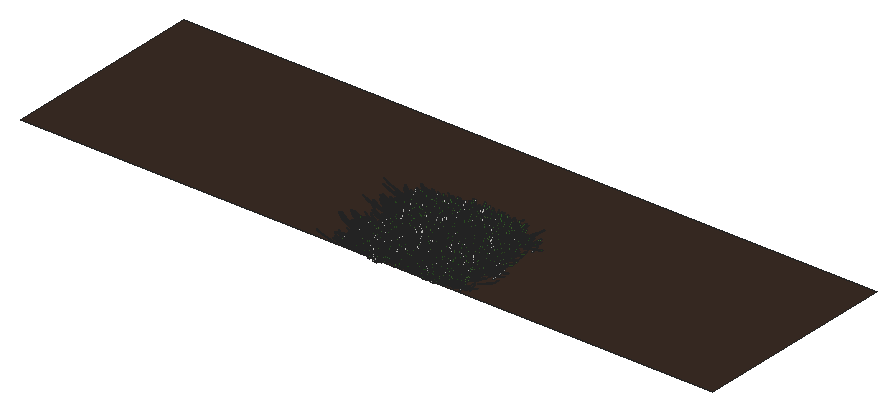
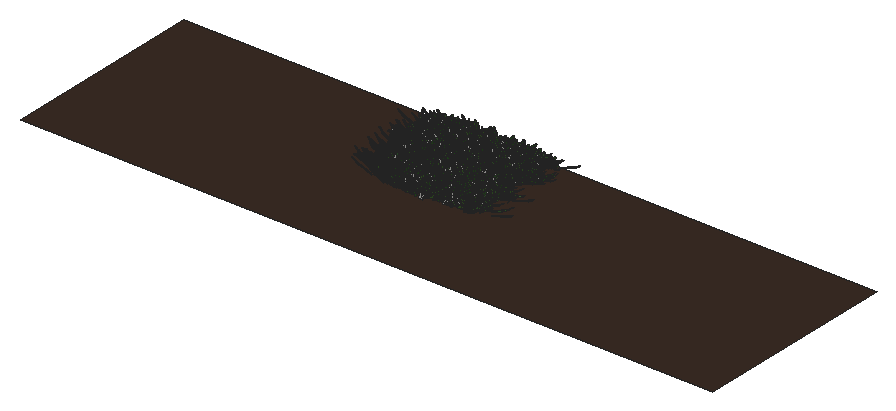
# SketchUp Ruby script. Lengths in inches.
U = 1.inch
M = Sketchup.active_model
def pt(a) = Geom::Point3d.new(a.map { |v| v * U })
def face(e, loops, mat)
  f = e.add_face(loops[0].map { |a| pt(a) })
  loops[1..].each { |l| e.add_face(l.map { |a| pt(a) }).erase! }
  f.material = f.back_material = mat if mat
  f
end
# faces: each face lists its corners as indices into pts; further lists are holes
def faces(e, pts, list, mat = nil) = list.each { |f| face(e, (f[0].is_a?(Array) ? f : [f]).map { |l| l.map { |i| pts[i] } }, mat) }
# xy, xz, yz: faces in a plane at the given z, y or x. An outline is a flat list of corners, or four numbers for a rectangle; further outlines are holes
def ring(l) = l.size == 4 ? [[l[0], l[1]], [l[2], l[1]], [l[2], l[3]], [l[0], l[3]]] : l.each_slice(2).to_a
def flat(e, list, mat, &to3) = list.each { |f| face(e, (f[0].is_a?(Array) ? f : [f]).map { |l| ring(l).map { |u, v| to3.(u, v) } }, mat) }
def xy(e, z, list, mat = nil) = flat(e, list, mat) { |x, y| [x, y, z] }
def xz(e, y, list, mat = nil) = flat(e, list, mat) { |x, z| [x, y, z] }
def yz(e, x, list, mat = nil) = flat(e, list, mat) { |y, z| [x, y, z] }
def lines(e, pts, list) = list.each { |a, b| e.add_line(pt(pts[a]), pt(pts[b])) }
# prism: a flat outline (further loops are holes) pulled along v
def prism(e, loops, v, mat = nil)
  f = face(e, loops, mat); d = Geom::Vector3d.new(v.map { |x| x * U })
  f.pushpull(f.normal.samedirection?(d) ? d.length : -d.length)
end
def box(e, o, s, mat = nil) = prism(e, [[o, [o[0] + s[0], o[1], o[2]], [o[0] + s[0], o[1] + s[1], o[2]], [o[0], o[1] + s[1], o[2]]]], [0, 0, s[2]], mat)
def at(x, y, z, deg = 0) = Geom::Transformation.translation(pt([x, y, z])) * Geom::Transformation.rotation(ORIGIN, Z_AXIS, deg.degrees)
def axes(o, x, y, z) = Geom::Transformation.new([*x, 0, *y, 0, *z, 0, *pt(o).to_a, 1])
def part(name) = M.definitions.add(name)
# library, detail: a bought-in or finely detailed component or shape, given as its bounding box
def library(name, o, s) = part(name).tap { |d| box(d.entities, o, s) }
def detail(e, o, s) = box(e.add_group.entities, o, s)
def put(e, d, t, mat = nil) = e.add_instance(d, t).tap { |i| i.material = mat if mat }
def group(e, t, mat = nil) = e.add_group.tap { |g| g.transformation = t; g.material = mat if mat }.entities
root = M.entities
M.materials.add("Material10").color = [48, 100, 38]
M.materials.add("Material3").color = [68, 110, 58]
M.materials.add("Material4").color = [48, 90, 38]
M.materials.add("Material5").color = [68, 110, 48]
M.materials.add("Material6").color = [48, 90, 48]
M.materials.add("Material7").color = [58, 110, 58]
M.materials.add("Material8").color = [58, 90, 38]
M.materials.add("Material9").color = [68, 100, 58]
M.materials.add("top-soil").color = [58, 44, 36]
c1 = part("grass00")
p = [[-0.6875,0.15,0],[-0.56,0.08,5.52],[-0.04,0.03,2.76],[0.48,-0.02,0],[0.35,-0.02,5.52],[-0.1,-0.14,5.52],
  [-0.12,0.65,8.37],[-0.42,0.65,8.37]]
faces(c1.entities,p,[[0,1,2,3],[3,2,4],[1,5,2],[5,4,2],[1,6,5],[4,5,6],[7,6,1]])
c2 = part("Group16\#1")
put(c2.entities,c1,axes([1.44,-0.61,-0.01],[0.05352,0.12609,0],[-0.10704,0.04543,0.07239],[0.06664,-0.02828,0.11628]),"Material6")
put(c2.entities,c1,axes([0.76,-0.15,-0.01],[0.04676,0.24062,0],[-0.23162,0.04501,0.06642],[0.0652,-0.01267,0.23595]),"Material3")
put(c2.entities,c1,axes([0.79,0.01,-0.01],[-0.00606,0.34651,0],[-0.34381,-0.00602,0.0432],[0.04319,0.00076,0.34386]))
put(c2.entities,c1,axes([1,0.23,-0.01],[-0.07192,0.31144,0],[-0.28722,-0.06632,0.1236],[0.12043,0.02781,0.29478]),"Material5")
put(c2.entities,c1,axes([1.66,0.77,-0.01],[-0.13828,0.29651,0],[-0.21551,-0.1005,0.22471],[0.20365,0.09498,0.23779]),"Material10")
put(c2.entities,c1,axes([0.6875,0.52,-0.01],[-0.18126,0.24051,0],[-0.22746,-0.17142,0.09788],[0.07817,0.05891,0.28481]),"Material5")
put(c2.entities,c1,axes([0.68,0.78,-0.01],[-0.215,0.18688,0],[-0.12385,-0.14248,0.21334],[0.13995,0.16101,0.18878]),"Material3")
put(c2.entities,c1,axes([0.56,1,-0.01],[-0.13756,0.07624,0],[-0.06159,-0.11112,0.0927],[0.04494,0.08108,0.12705]),"Material5")
put(c2.entities,c1,axes([0.2,0.64,-0.01],[-0.23729,0.07254,0],[-0.05711,-0.18681,0.153],[0.04473,0.14632,0.19535]),"Material10")
put(c2.entities,c1,axes([0.0625,0.72,-0.01],[-0.28874,0.02525,0],[-0.02179,-0.24916,0.14647],[0.01276,0.14591,0.25012]),"Material3")
put(c2.entities,c1,axes([-0.08,0.62,-0.01],[-0.34089,-0.04187,0],[0.03255,-0.26504,0.216],[-0.02633,0.21439,0.26703]),"Material10")
put(c2.entities,c1,axes([-0.34,0.98,-0.01],[-0.14314,-0.0493,0],[0.04397,-0.12769,0.06843],[-0.02228,0.0647,0.13505]),"Material10")
put(c2.entities,c1,axes([-0.87,1.45,-0.01],[-0.23488,-0.14114,0],[0.13761,-0.22901,0.06087],[-0.03135,0.05217,0.26717]))
put(c2.entities,c1,axes([-0.72,0.77,-0.01],[-0.14208,-0.13251,0],[0.07209,-0.0773,0.16301],[-0.11118,0.11922,0.1057]),"Material10")
put(c2.entities,c1,axes([-0.62,0.43,-0.01],[-0.14845,-0.21203,0],[0.18654,-0.13061,0.12304],[-0.10079,0.07057,0.22772]),"Material3")
put(c2.entities,c1,axes([-0.68,0.29,-0.01],[-0.13639,-0.32136,0],[0.31723,-0.13464,0.05579],[-0.05136,0.0218,0.34462]),"Material4")
put(c2.entities,c1,axes([-0.64,0.125,-0.01],[-0.0458,-0.23569,0],[0.22124,-0.043,0.08276],[-0.08124,0.01579,0.22538]),"Material7")
put(c2.entities,c1,axes([-1.6,-0.03,-0.01],[0.00576,-0.32897,0],[0.27526,0.00482,0.18018],[-0.18015,-0.00315,0.2753]),"Material5")
put(c2.entities,c1,axes([-1.36,-0.31,-0.01],[0.05718,-0.24765,0],[0.18172,0.04196,0.17267],[-0.16825,-0.03885,0.1865]),"Material10")
put(c2.entities,c1,axes([-1.54,-0.72,-0.01],[0.06537,-0.14017,0],[0.13555,0.06321,0.03939],[-0.0357,-0.01665,0.14956]))
put(c2.entities,c1,axes([-1.19,-0.9,-0.01],[0.09597,-0.12735,0],[0.11214,0.08451,0.07557],[-0.06035,-0.04548,0.14042]),"Material9")
put(c2.entities,c1,axes([-0.47,-0.54,-0.01],[0.11588,-0.10072,0],[0.0618,0.0711,0.12124],[-0.07953,-0.0915,0.0942]))
put(c2.entities,c1,axes([-0.47,-0.84,-0.01],[0.11927,-0.0661,0],[0.06603,0.11913,0.00646],[-0.00313,-0.00565,0.13621]),"Material5")
put(c2.entities,c1,axes([-0.38,-1.24,-0.01],[0.28037,-0.08571,0],[0.0618,0.20215,0.20315],[-0.05939,-0.19428,0.21139]),"Material9")
put(c2.entities,c1,axes([-0.06,-0.66,-0.01],[0.22719,-0.01987,0],[0.01247,0.14255,0.17758],[-0.01547,-0.17691,0.1431]),"Material8")
put(c2.entities,c1,axes([0.11,-0.89,-0.01],[0.14882,0.01828,0],[-0.01058,0.08611,0.12229],[0.01491,-0.12138,0.08676]),"Material6")
put(c2.entities,c1,axes([0.25,-0.72,-0.01],[0.20481,0.07053,0],[-0.06206,0.18022,0.10291],[0.03351,-0.0973,0.1906]),"Material6")
put(c2.entities,c1,axes([0.85,-1.42,-0.01],[0.16481,0.09904,0],[-0.09472,0.15762,0.05616],[0.02893,-0.04814,0.18389]),"Material5")
put(c2.entities,c1,axes([1.01,-1.09,-0.01],[0.21858,0.20385,0],[-0.17495,0.1876,0.15339],[0.10462,-0.11218,0.25652]),"Material10")
put(c2.entities,c1,axes([1.01,-0.71,-0.01],[0.08733,0.12473,0],[-0.06445,0.04512,0.13037],[0.1068,-0.07477,0.07867]),"Material6")
c3 = part("Group15\#1")
put(c3.entities,c2,at(0,0,0))
c4 = part("3darcstudiotree_grass00\#1")
put(c4.entities,c3,at(0,0,0))
xy(root,0,[[829.42,893.97,1095.56,972.71]],"top-soil")
put(root,c4,axes([956.87,929.05,0],[-4.13262,0.75948,0],[-2.24844,-0.76466,-0.00523],[-0.01922,-0.00654,1.47184]))
put(root,c4,axes([956.9,918.51,0],[-3.86969,0.48099,0],[-1.95079,-0.98092,-0.01143],[-0.02514,-0.01264,1.35283]))
put(root,c4,axes([955.9375,904.375,0],[3.86312,0.38228,0],[-1.39067,0.87833,-0.04887],[-0.14094,0.08902,1.85053]))
put(root,c4,axes([958,906.15,0],[-4.70177,-0.53336,0],[2.03054,-1.11874,-0.00153],[0.00375,-0.00206,1.82565]))
put(root,c4,axes([957.71,895.48,0],[-4.46822,-0.10581,0],[0.37585,-0.99198,-0.02721],[0.01358,-0.03584,1.31849]))
put(root,c4,axes([956.55,920.6875,0],[1.40657,1.03003,0],[-3.82031,0.32605,-0.04031],[-0.26799,0.02287,1.77227]))
put(root,c4,axes([957.67,927.64,0],[-3.92611,0.32664,0],[-1.54996,-1.16439,-0.02244],[-0.03763,-0.02827,1.62972]))
put(root,c4,axes([958.04,908.08,0],[0.29188,-1.2036,0],[4.4228,0.06704,-0.02606],[0.15802,0.0024,1.68211]))
put(root,c4,axes([957.74,903.37,0],[-2.65492,0.94025,0],[-3.53882,-0.62452,-0.04566],[-0.22738,-0.04013,1.65042]))
put(root,c4,axes([958.57,919.97,0],[4.17906,-0.20511,0],[0.89097,1.13456,-0.02697],[0.02876,0.03662,1.59996]))
put(root,c4,axes([961.06,909.17,0],[-4.41351,-0.36972,0],[1.24316,-0.9275,-0.02118],[0.04591,-0.03425,1.66873]))
put(root,c4,axes([961.57,905.5,0],[0.53348,-0.96081,0],[3.98331,0.13823,-0.0013],[0.00952,0.00033,1.85519]))
put(root,c4,axes([960.88,931.34,0],[-1.33514,1.21073,0],[-3.80153,-0.26201,-0.03305],[-0.17466,-0.01204,1.35106]))
put(root,c4,axes([961.51,918.44,0],[-2.22446,1.02155,0],[-4.2399,-0.57703,-0.05406],[-0.24223,-0.03297,1.53936]))
put(root,c4,axes([960.71,903.1,0],[1.18915,1.16091,0],[-4.66954,0.29894,-0.00469],[-0.02419,0.00155,1.60422]))
put(root,c4,axes([962.34,916.93,0],[-3.71937,0.41864,0],[-1.99025,-1.10514,-0.05685],[-0.1451,-0.08057,1.88376]))
put(root,c4,axes([961.62,896.51,0],[-0.88189,0.99912,0],[-4.57623,-0.25246,-0.05256],[-0.22927,-0.01265,1.30827]))
put(root,c4,axes([962.51,929.22,0],[1.87855,-0.80281,0],[3.39229,0.49612,-0.02347],[0.15921,0.02328,1.9305]))
put(root,c4,axes([963.25,915.51,0],[-0.60906,-0.96226,0],[5.07736,-0.20086,-0.05346],[0.24254,-0.00959,1.47567]))
put(root,c4,axes([962.55,900.55,0],[2.53298,-0.99579,0],[3.28482,0.52222,-0.04064],[0.20675,0.03287,1.46692]))
put(root,c4,axes([962.64,927.47,0],[2.73989,-0.60489,0],[2.55091,0.72216,-0.01409],[0.06366,0.01802,1.64399]))
put(root,c4,axes([962.89,907.07,0],[2.49365,-0.78367,0],[3.24543,0.64544,-0.01848],[0.08233,0.01637,1.47553]))
put(root,c4,axes([961.72,926.3,0],[4.4609,0.40125,0],[-1.29285,0.89834,-0.01256],[-0.03244,0.02254,1.82155]))
put(root,c4,axes([961.89,914.09,0],[2.4643,0.83625,0],[-3.57537,0.6585,-0.0323],[-0.14016,0.02581,1.496]))
put(root,c4,axes([962.58,922.3,0],[-1.53289,0.94847,0],[-3.89243,-0.39318,-0.02451],[-0.14378,-0.01452,1.66036]))
put(root,c4,axes([962.02,901.24,0],[3.75653,0.68918,0],[-2.16074,0.73611,-0.01519],[-0.05314,0.0181,1.34969]))
put(root,c4,axes([963.0625,898.6,0],[-1.332,1.0855,0],[-3.68359,-0.2825,-0.03727],[-0.23368,-0.01792,1.57911]))
put(root,c4,axes([962.375,910.39,0],[4.4023,0.31445,0],[-1.15221,1.00818,-0.01128],[-0.01903,0.01665,1.61003]))
put(root,c4,axes([962.73,912.25,0],[4.69374,-0.30667,0],[0.9938,0.95067,-0.02428],[0.04983,0.04767,1.99391]))
put(root,c4,axes([963.0625,924.35,0],[3.84654,0.1622,0],[-0.71389,1.05813,-0.03005],[-0.02875,0.04262,1.54341]))
put(root,c4,axes([963.62,895.32,0],[3.63097,-0.44195,0],[1.99155,1.02264,-0.02466],[0.05688,0.02921,1.49812]))
put(root,c4,axes([963.95,919.9,0],[-0.92615,0.92755,0],[-3.93926,-0.24583,-0.00012],[-0.00062,-0.00004,1.39497]))
put(root,c4,axes([964.31,930.63,0],[-1.66158,1.03755,0],[-3.61607,-0.36193,-0.01826],[-0.10251,-0.01026,1.47196]))
put(root,c4,axes([964.71,904.92,0],[3.53421,-0.66797,0],[2.63257,0.87056,-0.04167],[0.17144,0.05669,1.86151]))
put(root,c4,axes([966.3125,902.98,0],[-3.75679,-0.65225,0],[2.19929,-0.79171,-0.00375],[0.0162,-0.00583,1.82358]))
put(root,c4,axes([966.375,898.54,0],[-3.06353,-0.57111,0],[2.62826,-0.88115,-0.00029],[0.00107,-0.00036,1.69542]))
put(root,c4,axes([964.6,921.76,0],[4.12285,0.65297,0],[-2.36966,0.93513,-0.03414],[-0.094,0.03709,1.42377]))
put(root,c4,axes([966.47,908.08,0],[-4.09682,0.49001,0],[-2.11354,-1.10442,-0.05113],[-0.09658,-0.05047,1.33965]))
put(root,c4,axes([966.77,923.27,0],[3.22149,-0.77184,0],[3.4883,0.90996,-0.03986],[0.14566,0.038,1.66404]))
put(root,c4,axes([967.3,895.0625,0],[-3.99831,0.66373,0],[-2.79382,-1.05187,-0.05111],[-0.13772,-0.05185,1.53759]))
put(root,c4,axes([967.26,913.66,0],[-2.34879,0.82115,0],[-3.6953,-0.66061,-0.05929],[-0.24052,-0.043,1.41608]))
put(root,c4,axes([966.35,901.61,0],[2.86716,0.8976,0],[-2.85293,0.56956,-0.01421],[-0.0686,0.0137,1.40932]))
put(root,c4,axes([968.3,924.33,0],[-0.2584,-1.18473,0],[3.63618,-0.04957,-0.01049],[0.06761,-0.00092,1.4693]))
put(root,c4,axes([969.29,925.72,0],[-2.94405,-0.59903,0],[3.18153,-0.97726,-0.04334],[0.11663,-0.03583,1.34295]))
put(root,c4,axes([968.56,921.67,0],[2.52087,-0.77867,0],[3.74489,0.75773,-0.0352],[0.16916,0.03423,1.86157]))
put(root,c4,axes([969.625,919.6,0],[-4.25461,-0.72001,0],[2.67413,-0.98761,-0.04034],[0.12328,-0.04553,1.62559]))
put(root,c4,axes([967.35,906.34,0],[4.6579,0.46394,0],[-1.71341,1.07515,-0.01606],[-0.03179,0.01995,1.54782]))
put(root,c4,axes([967.68,918.33,0],[1.00242,0.87576,0],[-4.78791,0.34253,-0.02742],[-0.16399,0.01173,1.93645]))
put(root,c4,axes([967.95,912.02,0],[-0.10924,0.93543,0],[-4.47278,-0.03265,-0.00454],[-0.02701,-0.0002,1.66362]))
put(root,c4,axes([970.13,910.67,0],[-1.41075,-1.20737,0],[3.77402,-0.27561,-0.03009],[0.20256,-0.01479,1.72353]))
put(root,c4,axes([968.93,932.21,0],[4.18656,0.30844,0],[-1.02812,0.87218,-0.026],[-0.05159,0.04376,1.59572]))
put(root,c4,axes([970.61,929.97,0],[1.76759,-1.11088,0],[4.77436,0.4748,-0.04298],[0.2101,0.02089,1.68954]))
put(root,c4,axes([969.14,928.3,0],[4.47643,0.35496,0],[-1.36564,1.07638,-0.00141],[-0.00295,0.00232,1.95289]))
put(root,c4,axes([969.67,897.34,0],[0.44827,0.96887,0],[-3.98401,0.1152,-0.04522],[-0.2884,0.00834,1.60941]))
put(root,c4,axes([970.11,900.36,0],[-3.25483,0.8021,0],[-3.45367,-0.87591,-0.01243],[-0.05011,-0.01271,1.76595]))
put(root,c4,axes([970.125,927.02,0],[4.42338,-0.02191,0],[0.0799,1.00813,-0.01855],[0.00282,0.03561,1.93628]))
put(root,c4,axes([970.22,904.62,0],[1.52901,1.13008,0],[-3.97535,0.33617,-0.04556],[-0.25323,0.02141,1.53888]))
put(root,c4,axes([970.77,908.57,0],[4.69014,-0.44413,0],[1.55704,1.02768,-0.01068],[0.01805,0.01192,1.31138]))
put(root,c4,axes([970.73,917.21,0],[3.67709,0.37589,0],[-1.7272,1.05602,-0.03911],[-0.07805,0.04772,1.50402]))
put(root,c4,axes([972.84,911.08,0],[-2.16175,-1.00389,0],[3.8462,-0.51764,-0.02018],[0.12706,-0.0171,1.95264]))
put(root,c4,axes([972.78,921.2,0],[-2.62411,-0.67542,0],[2.85989,-0.69444,-0.02073],[0.09247,-0.02245,1.5494]))
put(root,c4,axes([970.64,915.15,0],[2.20682,1.15051,0],[-3.88825,0.46614,-0.00104],[-0.00548,0.00066,1.58037]))
put(root,c4,axes([973.375,919.47,0],[-3.73719,-0.68313,0],[2.19401,-0.75016,-0.03203],[0.15881,-0.0543,1.95145]))
put(root,c4,axes([972.48,895.74,0],[3.66888,-0.3039,0],[1.21402,0.91602,-0.03222],[0.07511,0.05667,1.78787]))
put(root,c4,axes([973.18,931.61,0],[2.44539,-0.83578,0],[3.06971,0.56135,-0.02877],[0.14565,0.02664,1.49076]))
put(root,c4,axes([974.78,916.98,0],[-2.07648,-1.05782,0],[4.05072,-0.49696,-0.01008],[0.05023,-0.00616,1.566]))
put(root,c4,axes([973.04,898.09,0],[0.11038,0.92839,0],[-4.43569,0.03296,-0.05613],[-0.30865,0.00229,1.5259]))
put(root,c4,axes([973.82,913.16,0],[3.30121,-0.61217,0],[2.52484,0.85098,-0.02804],[0.09819,0.03309,1.55696]))
put(root,c4,axes([972.97,897.5,0],[2.77049,0.67206,0],[-2.57835,0.66431,-0.00683],[-0.0359,0.00925,1.74693]))
put(root,c4,axes([974.64,928.97,0],[-4.82674,0.25422,0],[-0.88565,-1.05095,-0.00142],[-0.00177,-0.0021,1.63114]))
put(root,c4,axes([974.93,914.76,0],[-4.23216,-0.4101,0],[1.59131,-1.02639,-0.05586],[0.14093,-0.0909,1.92103]))
put(root,c4,axes([975.08,903.98,0],[0.04875,-0.97285,0],[3.90965,0.01225,-0.00992],[0.05364,0.00017,1.32167]))
put(root,c4,axes([974.77,930.45,0],[-4.10192,0.74973,0],[-2.75988,-0.94373,-0.03994],[-0.15914,-0.05442,1.97331]))
put(root,c4,axes([973.63,925.22,0],[5.03069,0.15304,0],[-0.59852,1.22962,-0.0359],[-0.02633,0.0541,1.88046]))
put(root,c4,axes([975.1,922.22,0],[1.61139,-0.92057,0],[3.30633,0.36172,-0.00213],[0.01129,0.00123,1.30651]))
put(root,c4,axes([976.33,899.66,0],[-2.89418,-0.78817,0],[3.81113,-0.87466,-0.02326],[0.09657,-0.02216,1.82249]))
put(root,c4,axes([975.73,901.89,0],[1.38566,-1.0009,0],[3.42279,0.29616,-0.00044],[0.00245,0.00021,1.32507]))
put(root,c4,axes([976.29,908.89,0],[-4.53149,-0.15613,0],[0.63638,-1.15439,-0.00876],[0.00543,-0.00985,1.32289]))
put(root,c4,axes([975.25,924.26,0],[-3.16538,1.0009,0],[-3.18179,-0.62891,-0.0043],[-0.02493,-0.00493,1.8735]))
put(root,c4,axes([974.26,918.5625,0],[2.46284,0.96083,0],[-4.30352,0.68944,-0.02786],[-0.14516,0.02326,1.9768]))
put(root,c4,axes([975.3125,902.73,0],[3.73009,0.22757,0],[-0.89297,0.9148,-0.01459],[-0.0258,0.02643,1.75568]))
put(root,c4,axes([975.39,933.45,0],[4.502,0.00283,0],[-0.01155,1.14774,-0.01268],[-0.0002,0.02022,1.83013]))
put(root,c4,axes([975.55,927.69,0],[5.05197,-0.08472,0],[0.33414,1.24538,-0.00473],[0.00152,0.00566,1.49489]))
put(root,c4,axes([975.46,906.08,0],[3.94341,0.43089,0],[-1.69112,0.9673,-0.01451],[-0.03524,0.02016,1.59989]))
put(root,c4,axes([976.66,907.86,0],[-1.02018,1.09305,0],[-3.99403,-0.23299,-0.02125],[-0.10851,-0.00633,1.34411]))
put(root,c4,axes([976.53,911.7,0],[1.6819,1.04129,0],[-4.31148,0.43525,-0.05886],[-0.25156,0.0254,1.33951]))
put(root,c4,axes([979,907.47,0],[-2.51512,-0.77135,0],[3.2397,-0.66023,-0.00371],[0.01648,-0.00336,1.4993]))
put(root,c4,axes([978.92,932.04,0],[-2.73008,-0.65952,0],[3.11842,-0.80679,-0.03177],[0.14282,-0.03695,1.8145]))
put(root,c4,axes([978.71,911.81,0],[-3.14493,1.01166,0],[-3.08712,-0.59981,-0.03149],[-0.13615,-0.02645,1.33797]))
put(root,c4,axes([978.65,906,0],[-3.00004,0.96775,0],[-4.04392,-0.78352,-0.03455],[-0.13505,-0.02617,1.58129]))
put(root,c4,axes([980.23,925.59,0],[-3.06002,-0.4895,0],[1.9457,-0.7602,-0.02395],[0.07981,-0.03118,1.39534]))
put(root,c4,axes([978.93,899.53,0],[4.73916,-0.2961,0],[1.22977,1.23018,-0.03338],[0.03516,0.03517,1.37691]))
put(root,c4,axes([979.23,917.7,0],[3.7155,-0.16397,0],[0.83101,1.17689,-0.03701],[0.04274,0.06052,1.98432]))
put(root,c4,axes([979.17,923.77,0],[1.11685,0.86772,0],[-3.58583,0.28846,-0.0339],[-0.24805,0.01995,1.80984]))
put(root,c4,axes([979.66,904.36,0],[3.47383,0.27183,0],[-1.15707,0.92418,-0.01935],[-0.04591,0.03667,1.92273]))
put(root,c4,axes([980,916.15,0],[3.76768,-0.14266,0],[0.7468,1.23267,-0.05863],[0.04677,0.07719,1.66018]))
put(root,c4,axes([980.89,930.68,0],[-2.77251,0.84183,0],[-3.16826,-0.65216,-0.04557],[-0.25419,-0.05232,1.85346]))
put(root,c4,axes([981.72,898.66,0],[-4.19889,-0.35497,0],[1.51882,-1.12287,-0.06149],[0.11991,-0.08865,1.80385]))
put(root,c4,axes([981.83,915.64,0],[-2.26034,-0.95612,0],[4.04504,-0.59768,-0.04139],[0.22409,-0.03311,1.84708]))
put(root,c4,axes([979.86,922.38,0],[2.33279,0.76327,0],[-3.38254,0.64613,-0.0123],[-0.05875,0.01122,1.59876]))
put(root,c4,axes([982.14,926.78,0],[-4.70227,-0.09202,0],[0.37427,-1.19528,-0.05117],[0.02052,-0.06554,1.54048]))
put(root,c4,axes([980.64,895.3,0],[4.48386,0.0868,0],[-0.3465,1.11875,-0.0417],[-0.02197,0.07094,1.91485]))
put(root,c4,axes([982.12,913.15,0],[-4.35252,0.40027,0],[-1.39021,-0.94482,-0.04924],[-0.13398,-0.09105,1.98345]))
put(root,c4,axes([980.73,921.54,0],[5.08464,-0.02369,0],[0.09161,1.22889,-0.03615],[0.00341,0.04568,1.55355]))
put(root,c4,axes([980.56,896.91,0],[3.96051,0.53501,0],[-2.37184,1.09738,-0.05913],[-0.12576,0.05819,1.39517]))
put(root,c4,axes([982.11,901.49,0],[-3.78367,0.13136,0],[-0.66281,-1.19321,-0.02154],[-0.01411,-0.0254,1.4342]))
put(root,c4,axes([982.54,933.01,0],[-3.49013,-0.33538,0],[1.59635,-1.03827,-0.04802],[0.0959,-0.06237,1.54794]))
put(root,c4,axes([981.44,902.64,0],[1.46709,1.05523,0],[-3.46881,0.30142,-0.01128],[-0.08445,0.00734,1.81963]))
put(root,c4,axes([982.06,909.6,0],[-0.91674,0.93893,0],[-3.90242,-0.23814,-0.03757],[-0.1913,-0.01167,1.3158]))
put(root,c4,axes([982.89,911.17,0],[3.37683,-0.41478,0],[2.02863,1.03221,-0.05746],[0.17419,0.08863,1.97658]))
put(root,c4,axes([982.77,920.2,0],[1.70448,0.82052,0],[-3.56359,0.46267,-0.04821],[-0.23323,0.03028,1.36797]))
put(root,c4,axes([982.92,928.93,0],[0.92537,0.88194,0],[-4.41154,0.2893,-0.05161],[-0.26626,0.01746,1.52021]))
put(root,c4,axes([985.33,915,0],[-4.05837,-0.6928,0],[2.05635,-0.75288,-0.01838],[0.08227,-0.03012,1.80866]))
put(root,c4,axes([985.35,926.18,0],[0.10765,-0.97031,0],[3.90714,0.02709,-0.00183],[0.01108,0.00008,1.48199]))
put(root,c4,axes([985.01,902,0],[2.38443,-0.79485,0],[3.89504,0.73029,-0.03529],[0.12587,0.0236,1.35654]))
put(root,c4,axes([986.03,910.72,0],[-4.4757,-0.23245,0],[1.02085,-1.22848,-0.02537],[0.03005,-0.03616,1.82613]))
put(root,c4,axes([985.66,918.3125,0],[-4.25208,0.35979,0],[-1.19702,-0.88418,-0.02484],[-0.06716,-0.04961,1.96802]))
put(root,c4,axes([985.97,904.6,0],[-4.39783,0.19091,0],[-0.81712,-1.17645,-0.05401],[-0.04088,-0.05885,1.3206]))
put(root,c4,axes([985.36,907.9375,0],[-2.10693,0.77136,0],[-3.00017,-0.51217,-0.01899],[-0.12155,-0.02075,1.75992]))
put(root,c4,axes([984.63,895.11,0],[-0.15623,0.94532,0],[-4.49196,-0.0464,-0.00296],[-0.0156,-0.00016,1.47961]))
put(root,c4,axes([984.92,911.65,0],[-0.40598,1.27803,0],[-4.68179,-0.09295,-0.01448],[-0.07168,-0.00142,1.45727]))
put(root,c4,axes([985.15,931.66,0],[4.58397,0.20442,0],[-0.68449,0.9593,-0.04495],[-0.06411,0.08985,1.97854]))
put(root,c4,axes([987.43,913.22,0],[-0.75592,-0.93689,0],[4.57802,-0.23086,-0.04603],[0.25634,-0.01293,1.65834]))
put(root,c4,axes([985.91,896.53,0],[4.03398,0.31007,0],[-1.40845,1.14523,-0.02064],[-0.02977,0.02421,1.46981]))
put(root,c4,axes([987.375,922.36,0],[-4.15465,0.6663,0],[-2.35272,-0.91688,-0.01729],[-0.05585,-0.02177,1.62898]))
put(root,c4,axes([988.08,902.5625,0],[-3.83717,-0.19208,0],[0.9693,-1.21021,-0.02406],[0.02351,-0.02935,1.53532]))
put(root,c4,axes([988.38,927.27,0],[-4.91779,-0.19601,0],[0.6703,-1.05111,-0.05098],[0.05043,-0.07908,1.67187]))
put(root,c4,axes([986.8,919.98,0],[4.59957,-0.09357,0],[0.3643,1.11918,-0.01977],[0.00913,0.02806,1.59866]))
put(root,c4,axes([988.1875,921.08,0],[-4.94513,0.23867,0],[-0.82278,-1.06546,-0.00152],[-0.0015,-0.00195,1.41339]))
put(root,c4,axes([987.03,916.1,0],[-1.34706,1.11667,0],[-4.07742,-0.30742,-0.01363],[-0.0693,-0.00522,1.41312]))
put(root,c4,axes([987.77,898.66,0],[-2.30928,0.69091,0],[-3.20293,-0.66909,-0.03387],[-0.15372,-0.03211,1.54303]))
put(root,c4,axes([987.6,900.16,0],[3.65365,-0.40447,0],[2.03299,1.14777,-0.04981],[0.11291,0.06375,1.75709]))
put(root,c4,axes([987.25,924.26,0],[2.59051,0.81942,0],[-3.35986,0.66386,-0.02315],[-0.11156,0.02204,1.64391]))
put(root,c4,axes([987.12,930.36,0],[2.96025,0.64544,0],[-3.39185,0.97228,-0.01764],[-0.06278,0.018,1.74631]))
put(root,c4,axes([988.54,909.02,0],[3.11892,-0.94287,0],[3.04529,0.6296,-0.04304],[0.23637,0.04887,1.76026]))
put(root,c4,axes([987.93,905.59,0],[0.28426,1.04534,0],[-4.32493,0.07351,-0.02807],[-0.13623,0.00232,1.3177]))
put(root,c4,axes([990.79,895.79,0],[-2.81125,-0.60832,0],[3.02098,-0.87256,-0.00422],[0.01275,-0.00368,1.33295]))
put(root,c4,axes([988.9,928.71,0],[3.79286,0.40503,0],[-1.76539,1.03325,-0.00364],[-0.00998,0.00584,1.96053]))
put(root,c4,axes([992.02,927.51,0],[-2.87569,-1.00726,0],[3.7505,-0.66922,-0.01802],[0.06852,-0.01223,1.345]))
put(root,c4,axes([991.48,921.4375,0],[-3.91989,0.02908,0],[-0.12642,-1.06499,-0.02538],[-0.00493,-0.04149,1.74242]))
put(root,c4,axes([990.67,906.02,0],[-2.30919,0.93176,0],[-3.9041,-0.60472,-0.01218],[-0.05759,-0.00892,1.59607]))
put(root,c4,axes([991.45,901.8125,0],[3.80375,-0.52233,0],[2.25643,1.02699,-0.02691],[0.07906,0.03598,1.78778]))
put(root,c4,axes([992.84,896.93,0],[-1.71233,-0.84239,0],[3.99342,-0.50734,-0.00876],[0.04062,-0.00516,1.45672]))
put(root,c4,axes([993.1,907.49,0],[-3.48158,-0.93813,0],[3.46536,-0.80378,-0.01209],[0.04881,-0.01132,1.62724]))
put(root,c4,axes([993.17,910.38,0],[-2.81575,-0.88554,0],[3.65217,-0.7258,-0.01168],[0.04216,-0.00838,1.34439]))
put(root,c4,axes([991.32,918.04,0],[-0.1762,1.09115,0],[-4.68185,-0.04725,-0.04298],[-0.27686,-0.00279,1.88799]))
put(root,c4,axes([993.23,913.42,0],[-3.80607,-0.23651,0],[1.18989,-1.19677,-0.01735],[0.0231,-0.02323,1.70162]))
